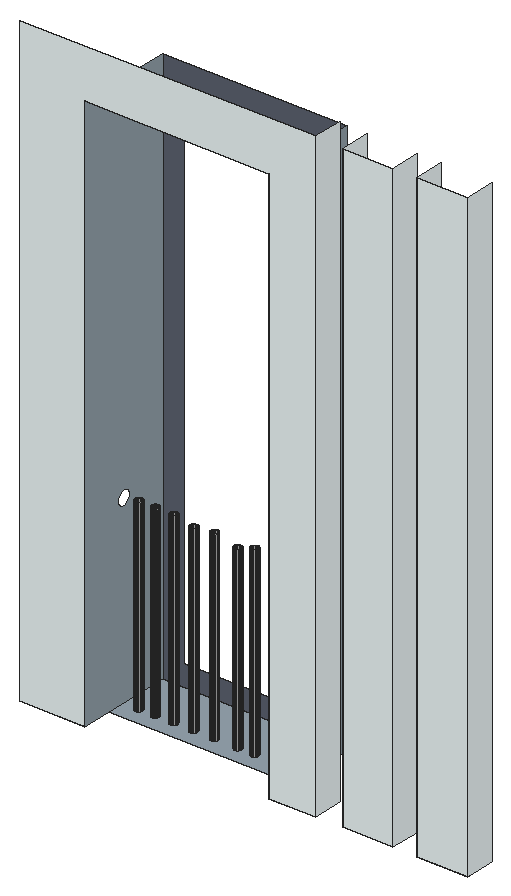
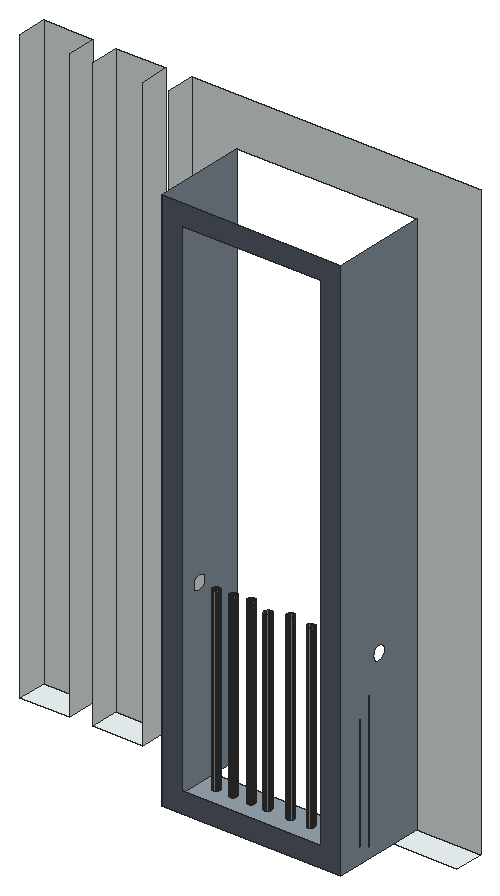
# SketchUp Ruby script. Lengths in inches.
U = 1.inch
M = Sketchup.active_model
def pt(a) = Geom::Point3d.new(a.map { |v| v * U })
def face(e, loops, mat)
  f = e.add_face(loops[0].map { |a| pt(a) })
  loops[1..].each { |l| e.add_face(l.map { |a| pt(a) }).erase! }
  f.material = f.back_material = mat if mat
  f
end
# faces: each face lists its corners as indices into pts; further lists are holes
def faces(e, pts, list, mat = nil) = list.each { |f| face(e, (f[0].is_a?(Array) ? f : [f]).map { |l| l.map { |i| pts[i] } }, mat) }
# xy, xz, yz: faces in a plane at the given z, y or x. An outline is a flat list of corners, or four numbers for a rectangle; further outlines are holes
def ring(l) = l.size == 4 ? [[l[0], l[1]], [l[2], l[1]], [l[2], l[3]], [l[0], l[3]]] : l.each_slice(2).to_a
def flat(e, list, mat, &to3) = list.each { |f| face(e, (f[0].is_a?(Array) ? f : [f]).map { |l| ring(l).map { |u, v| to3.(u, v) } }, mat) }
def xy(e, z, list, mat = nil) = flat(e, list, mat) { |x, y| [x, y, z] }
def xz(e, y, list, mat = nil) = flat(e, list, mat) { |x, z| [x, y, z] }
def yz(e, x, list, mat = nil) = flat(e, list, mat) { |y, z| [x, y, z] }
def lines(e, pts, list) = list.each { |a, b| e.add_line(pt(pts[a]), pt(pts[b])) }
# prism: a flat outline (further loops are holes) pulled along v
def prism(e, loops, v, mat = nil)
  f = face(e, loops, mat); d = Geom::Vector3d.new(v.map { |x| x * U })
  f.pushpull(f.normal.samedirection?(d) ? d.length : -d.length)
end
def box(e, o, s, mat = nil) = prism(e, [[o, [o[0] + s[0], o[1], o[2]], [o[0] + s[0], o[1] + s[1], o[2]], [o[0], o[1] + s[1], o[2]]]], [0, 0, s[2]], mat)
def at(x, y, z, deg = 0) = Geom::Transformation.translation(pt([x, y, z])) * Geom::Transformation.rotation(ORIGIN, Z_AXIS, deg.degrees)
def axes(o, x, y, z) = Geom::Transformation.new([*x, 0, *y, 0, *z, 0, *pt(o).to_a, 1])
def part(name) = M.definitions.add(name)
# library, detail: a bought-in or finely detailed component or shape, given as its bounding box
def library(name, o, s) = part(name).tap { |d| box(d.entities, o, s) }
def detail(e, o, s) = box(e.add_group.entities, o, s)
def put(e, d, t, mat = nil) = e.add_instance(d, t).tap { |i| i.material = mat if mat }
def group(e, t, mat = nil) = e.add_group.tap { |g| g.transformation = t; g.material = mat if mat }.entities
root = M.entities
M.materials.add("[Color M03]").color = [170, 170, 170]
M.materials.add("[Formica Laminate Dark]").color = [95, 101, 114]
M.materials.add("[Terrazzo Light Blue]").color = [151, 165, 175]
M.materials.add("[White Subway Tile]").color = [243, 252, 253]
xy(root,1217.33,[[1131.58,820.58,1130.43,820.73,1129.36,821.17,1128.44,821.88,1127.74,822.8,1127.29,823.87,1127.14,825.02,1127.29,826.17,1127.74,827.24,1128.44,828.15,1129.36,828.86,1130.43,829.3,1131.58,829.45,1132.73,829.3,1133.8,828.86,1134.72,828.15,1135.42,827.24,1135.87,826.17,1136.02,825.02,1135.87,823.87,1135.42,822.8,1134.72,821.88,1133.8,821.17,1132.73,820.73],[1151.52,820.58,1150.37,820.73,1149.3,821.17,1148.38,821.88,1147.67,822.8,1147.23,823.87,1147.08,825.02,1147.23,826.17,1147.67,827.24,1148.38,828.15,1149.3,828.86,1150.37,829.3,1151.52,829.45,1152.67,829.3,1153.74,828.86,1154.65,828.15,1155.36,827.24,1155.8,826.17,1155.95,825.02,1155.8,823.87,1155.36,822.8,1154.65,821.88,1153.74,821.17,1152.67,820.73],[1173.58,820.58,1172.43,820.73,1171.36,821.17,1170.44,821.88,1169.74,822.8,1169.29,823.87,1169.14,825.02,1169.29,826.17,1169.74,827.24,1170.44,828.15,1171.36,828.86,1172.43,829.3,1173.58,829.45,1174.73,829.3,1175.8,828.86,1176.72,828.15,1177.42,827.24,1177.87,826.17,1178.02,825.02,1177.87,823.87,1177.42,822.8,1176.72,821.88,1175.8,821.17,1174.73,820.73],[1197.58,820.58,1196.43,820.73,1195.36,821.17,1194.44,821.88,1193.74,822.8,1193.29,823.87,1193.14,825.02,1193.29,826.17,1193.74,827.24,1194.44,828.15,1195.36,828.86,1196.43,829.3,1197.58,829.45,1198.73,829.3,1199.8,828.86,1200.72,828.15,1201.42,827.24,1201.87,826.17,1202.02,825.02,1201.87,823.87,1201.42,822.8,1200.72,821.88,1199.8,821.17,1198.73,820.73],[1222.58,820.58,1221.43,820.73,1220.36,821.17,1219.44,821.88,1218.74,822.8,1218.29,823.87,1218.14,825.02,1218.29,826.17,1218.74,827.24,1219.44,828.15,1220.36,828.86,1221.43,829.3,1222.58,829.45,1223.73,829.3,1224.8,828.86,1225.72,828.15,1226.42,827.24,1226.87,826.17,1227.02,825.02,1226.87,823.87,1226.42,822.8,1225.72,821.88,1224.8,821.17,1223.73,820.73],
  [1250.58,820.58,1249.43,820.73,1248.36,821.17,1247.44,821.88,1246.74,822.8,1246.29,823.87,1246.14,825.02,1246.29,826.17,1246.74,827.24,1247.44,828.15,1248.36,828.86,1249.43,829.3,1250.58,829.45,1251.73,829.3,1252.8,828.86,1253.72,828.15,1254.42,827.24,1254.87,826.17,1255.02,825.02,1254.87,823.87,1254.42,822.8,1253.72,821.88,1252.8,821.17,1251.73,820.73],[1271.08,820.58,1269.93,820.73,1268.86,821.17,1267.94,821.88,1267.24,822.8,1266.79,823.87,1266.64,825.02,1266.79,826.17,1267.24,827.24,1267.94,828.15,1268.86,828.86,1269.93,829.3,1271.08,829.45,1272.23,829.3,1273.3,828.86,1274.22,828.15,1274.92,827.24,1275.37,826.17,1275.52,825.02,1275.37,823.87,1274.92,822.8,1274.22,821.88,1273.3,821.17,1272.23,820.73],[1292.95,820.58,1291.81,820.73,1290.74,821.17,1289.82,821.88,1289.11,822.8,1288.67,823.87,1288.52,825.02,1288.67,826.17,1289.11,827.24,1289.82,828.15,1290.74,828.86,1291.81,829.3,1292.95,829.45,1294.1,829.3,1295.17,828.86,1296.09,828.15,1296.8,827.24,1297.24,826.17,1297.39,825.02,1297.24,823.87,1296.8,822.8,1296.09,821.88,1295.17,821.17,1294.1,820.73],[1314.2,820.58,1313.06,820.73,1311.99,821.17,1311.07,821.88,1310.36,822.8,1309.92,823.87,1309.77,825.02,1309.92,826.17,1310.36,827.24,1311.07,828.15,1311.99,828.86,1313.06,829.3,1314.2,829.45,1315.35,829.3,1316.42,828.86,1317.34,828.15,1318.05,827.24,1318.49,826.17,1318.64,825.02,1318.49,823.87,1318.05,822.8,1317.34,821.88,1316.42,821.17,1315.35,820.73]])
xy(root,1217.33,[[[1113.04,803.71,1334.04,884.27],[1131.58,820.58,1130.43,820.73,1129.36,821.17,1128.44,821.88,1127.74,822.8,1127.29,823.87,1127.14,825.02,1127.29,826.17,1127.74,827.24,1128.44,828.15,1129.36,828.86,1130.43,829.3,1131.58,829.45,1132.73,829.3,1133.8,828.86,1134.72,828.15,1135.42,827.24,1135.87,826.17,1136.02,825.02,1135.87,823.87,1135.42,822.8,1134.72,821.88,1133.8,821.17,1132.73,820.73],[1314.2,820.58,1313.06,820.73,1311.99,821.17,1311.07,821.88,1310.36,822.8,1309.92,823.87,1309.77,825.02,1309.92,826.17,1310.36,827.24,1311.07,828.15,1311.99,828.86,1313.06,829.3,1314.2,829.45,1315.35,829.3,1316.42,828.86,1317.34,828.15,1318.05,827.24,1318.49,826.17,1318.64,825.02,1318.49,823.87,1318.05,822.8,1317.34,821.88,1316.42,821.17,1315.35,820.73],[1151.52,820.58,1150.37,820.73,1149.3,821.17,1148.38,821.88,1147.67,822.8,1147.23,823.87,1147.08,825.02,1147.23,826.17,1147.67,827.24,1148.38,828.15,1149.3,828.86,1150.37,829.3,1151.52,829.45,1152.67,829.3,1153.74,828.86,1154.65,828.15,1155.36,827.24,1155.8,826.17,1155.95,825.02,1155.8,823.87,1155.36,822.8,1154.65,821.88,1153.74,821.17,1152.67,820.73],[1292.95,820.58,1291.81,820.73,1290.74,821.17,1289.82,821.88,1289.11,822.8,1288.67,823.87,1288.52,825.02,1288.67,826.17,1289.11,827.24,1289.82,828.15,1290.74,828.86,1291.81,829.3,1292.95,829.45,1294.1,829.3,1295.17,828.86,1296.09,828.15,1296.8,827.24,1297.24,826.17,1297.39,825.02,1297.24,823.87,1296.8,822.8,1296.09,821.88,1295.17,821.17,1294.1,820.73],[1173.58,820.58,1172.43,820.73,1171.36,821.17,1170.44,821.88,1169.74,822.8,1169.29,823.87,1169.14,825.02,1169.29,826.17,1169.74,827.24,1170.44,828.15,1171.36,828.86,1172.43,829.3,1173.58,829.45,1174.73,829.3,1175.8,828.86,1176.72,828.15,1177.42,827.24,1177.87,826.17,1178.02,825.02,1177.87,823.87,1177.42,822.8,1176.72,821.88,1175.8,821.17,1174.73,820.73],[1271.08,820.58,1269.93,820.73,1268.86,821.17,1267.94,821.88,1267.24,822.8,1266.79,823.87,1266.64,825.02,1266.79,826.17,1267.24,827.24,1267.94,828.15,1268.86,828.86,1269.93,829.3,1271.08,829.45,1272.23,829.3,1273.3,828.86,1274.22,828.15,1274.92,827.24,1275.37,826.17,1275.52,825.02,1275.37,823.87,1274.92,822.8,1274.22,821.88,1273.3,821.17,1272.23,820.73],[1197.58,820.58,1196.43,820.73,1195.36,821.17,1194.44,821.88,1193.74,822.8,1193.29,823.87,1193.14,825.02,1193.29,826.17,1193.74,827.24,1194.44,828.15,1195.36,828.86,1196.43,829.3,1197.58,829.45,1198.73,829.3,1199.8,828.86,1200.72,828.15,1201.42,827.24,1201.87,826.17,1202.02,825.02,1201.87,823.87,1201.42,822.8,1200.72,821.88,1199.8,821.17,1198.73,820.73],[1250.58,820.58,1249.43,820.73,1248.36,821.17,1247.44,821.88,1246.74,822.8,1246.29,823.87,1246.14,825.02,1246.29,826.17,1246.74,827.24,1247.44,828.15,1248.36,828.86,1249.43,829.3,1250.58,829.45,1251.73,829.3,1252.8,828.86,1253.72,828.15,1254.42,827.24,1254.87,826.17,1255.02,825.02,1254.87,823.87,1254.42,822.8,1253.72,821.88,1252.8,821.17,1251.73,820.73],[1222.58,820.58,1221.43,820.73,1220.36,821.17,1219.44,821.88,1218.74,822.8,1218.29,823.87,1218.14,825.02,1218.29,826.17,1218.74,827.24,1219.44,828.15,1220.36,828.86,1221.43,829.3,1222.58,829.45,1223.73,829.3,1224.8,828.86,1225.72,828.15,1226.42,827.24,1226.87,826.17,1227.02,825.02,1226.87,823.87,1226.42,822.8,1225.72,821.88,1224.8,821.17,1223.73,820.73]]],"[Terrazzo Light Blue]")
xy(root,1217.33,[[1034.97,767.89,1113.04,803.71],[1334.04,767.89,1389.66,803.71]],"[White Subway Tile]")
xy(root,1217.36,[[1421.94,767.89,1482.63,803.71],[1511.44,767.89,1572.13,803.71]],"[White Subway Tile]")
xz(root,767.89,[[1034.97,1217.33,1113.04,1217.33,1113.04,1889.95,1334.04,1889.95,1334.04,1217.33,1389.66,1217.33,1389.66,1949.53,1034.97,1949.53],[1421.94,1217.36,1482.63,1947.36],[1511.44,1217.36,1572.13,1947.36]],"[White Subway Tile]")
xz(root,884.27,[[[1113.04,1217.33,1334.04,1889.95],[1137.95,1242.25,1309.12,1865.04]]],"[Formica Laminate Dark]")
yz(root,1113.04,[[[767.89,1217.33,884.27,1889.95],[826.07,1428.86,823.76,1429.16,821.6,1430.06,819.75,1431.48,818.33,1433.33,817.4375,1435.48,817.13,1437.8,817.4375,1440.11,818.33,1442.27,819.75,1444.12,821.6,1445.54,823.76,1446.43,826.07,1446.73,828.38,1446.43,830.54,1445.54,832.39,1444.12,833.8125,1442.27,834.7,1440.11,835.01,1437.8,834.7,1435.48,833.8125,1433.33,832.39,1431.48,830.54,1430.06,828.38,1429.16]]],"[Terrazzo Light Blue]")
yz(root,1334.04,[[[767.89,1217.33,884.27,1889.95],[826.07,1428.86,828.38,1429.16,830.54,1430.06,832.39,1431.48,833.8125,1433.33,834.7,1435.48,835.01,1437.8,834.7,1440.11,833.8125,1442.27,832.39,1444.12,830.54,1445.54,828.38,1446.43,826.07,1446.73,823.76,1446.43,821.6,1445.54,819.75,1444.12,818.33,1442.27,817.4375,1440.11,817.13,1437.8,817.4375,1435.48,818.33,1433.33,819.75,1431.48,821.6,1430.06,823.76,1429.16]]],"[Terrazzo Light Blue]")
yz(root,1389.66,[[767.89,1217.33,803.71,1949.53]],"[White Subway Tile]")
yz(root,1421.94,[[767.89,1217.36,803.71,1947.36]],"[White Subway Tile]")
yz(root,1482.63,[[767.89,1217.36,803.71,1947.36]],"[White Subway Tile]")
yz(root,1511.44,[[767.89,1217.36,803.71,1947.36]],"[White Subway Tile]")
yz(root,1572.13,[[767.89,1217.36,803.71,1947.36]],"[White Subway Tile]")
p = [[1130.43,820.73,1217.33],[1131.58,820.58,1217.33],[1131.58,820.58,1442.27],[1130.43,820.73,1442.27],[1132.73,820.73,1217.33],[1132.73,820.73,1442.27],
  [1150.37,820.73,1217.33],[1151.52,820.58,1217.33],[1151.52,820.58,1442.27],[1150.37,820.73,1442.27],[1152.67,820.73,1217.33],[1152.67,820.73,1442.27],
  [1172.43,820.73,1217.33],[1173.58,820.58,1217.33],[1173.58,820.58,1442.27],[1172.43,820.73,1442.27],[1174.73,820.73,1217.33],[1174.73,820.73,1442.27],
  [1196.43,820.73,1217.33],[1197.58,820.58,1217.33],[1197.58,820.58,1437.08],[1196.43,820.73,1437.08],[1198.73,820.73,1217.33],[1198.73,820.73,1437.08],
  [1221.43,820.73,1217.33],[1222.58,820.58,1217.33],[1222.58,820.58,1440.11],[1221.43,820.73,1440.11],[1223.73,820.73,1217.33],[1223.73,820.73,1440.11],
  [1249.43,820.73,1217.33],[1250.58,820.58,1217.33],[1250.58,820.58,1433.45],[1249.43,820.73,1433.45],[1251.73,820.73,1217.33],[1251.73,820.73,1433.45],
  [1269.93,820.73,1217.33],[1271.08,820.58,1217.33],[1271.08,820.58,1440.11],[1269.93,820.73,1440.11],[1272.23,820.73,1217.33],[1272.23,820.73,1440.11],
  [1291.81,820.73,1217.33],[1292.95,820.58,1217.33],[1292.95,820.58,1437.8],[1291.81,820.73,1437.8],[1294.1,820.73,1217.33],[1294.1,820.73,1437.8],
  [1313.06,820.73,1217.33],[1314.2,820.58,1217.33],[1314.2,820.58,1436.77],[1313.06,820.73,1436.77],[1315.35,820.73,1217.33],[1315.35,820.73,1436.77],
  [1129.36,821.17,1217.33],[1129.36,821.17,1442.27],[1133.8,821.17,1217.33],[1133.8,821.17,1442.27],[1149.3,821.17,1217.33],[1149.3,821.17,1442.27],
  [1153.74,821.17,1217.33],[1153.74,821.17,1442.27],[1171.36,821.17,1217.33],[1171.36,821.17,1442.27],[1175.8,821.17,1217.33],[1175.8,821.17,1442.27],
  [1195.36,821.17,1217.33],[1195.36,821.17,1437.08],[1199.8,821.17,1217.33],[1199.8,821.17,1437.08],[1220.36,821.17,1217.33],[1220.36,821.17,1440.11],
  [1224.8,821.17,1217.33],[1224.8,821.17,1440.11],[1248.36,821.17,1217.33],[1248.36,821.17,1433.45],[1252.8,821.17,1217.33],[1252.8,821.17,1433.45],
  [1268.86,821.17,1217.33],[1268.86,821.17,1440.11],[1273.3,821.17,1217.33],[1273.3,821.17,1440.11],[1290.74,821.17,1217.33],[1290.74,821.17,1437.8],
  [1295.17,821.17,1217.33],[1295.17,821.17,1437.8],[1311.99,821.17,1217.33],[1311.99,821.17,1436.77],[1316.42,821.17,1217.33],[1316.42,821.17,1436.77],
  [1128.44,821.88,1217.33],[1128.44,821.88,1442.27],[1134.72,821.88,1217.33],[1134.72,821.88,1442.27],[1148.38,821.88,1217.33],[1148.38,821.88,1442.27],
  [1154.65,821.88,1217.33],[1154.65,821.88,1442.27],[1170.44,821.88,1217.33],[1170.44,821.88,1442.27],[1176.72,821.88,1217.33],[1176.72,821.88,1442.27],
  [1194.44,821.88,1217.33],[1194.44,821.88,1437.08],[1200.72,821.88,1217.33],[1200.72,821.88,1437.08],[1219.44,821.88,1217.33],[1219.44,821.88,1440.11],
  [1225.72,821.88,1217.33],[1225.72,821.88,1440.11],[1247.44,821.88,1217.33],[1247.44,821.88,1433.45],[1253.72,821.88,1217.33],[1253.72,821.88,1433.45],
  [1267.94,821.88,1217.33],[1267.94,821.88,1440.11],[1274.22,821.88,1217.33],[1274.22,821.88,1440.11],[1289.82,821.88,1217.33],[1289.82,821.88,1437.8],
  [1296.09,821.88,1217.33],[1296.09,821.88,1437.8],[1311.07,821.88,1217.33],[1311.07,821.88,1436.77],[1317.34,821.88,1217.33],[1317.34,821.88,1436.77],
  [1127.74,822.8,1217.33],[1127.74,822.8,1442.27],[1135.42,822.8,1217.33],[1135.42,822.8,1442.27],[1147.67,822.8,1217.33],[1147.67,822.8,1442.27],
  [1155.36,822.8,1217.33],[1155.36,822.8,1442.27],[1169.74,822.8,1217.33],[1169.74,822.8,1442.27],[1177.42,822.8,1217.33],[1177.42,822.8,1442.27],
  [1193.74,822.8,1217.33],[1193.74,822.8,1437.08],[1201.42,822.8,1217.33],[1201.42,822.8,1437.08],[1218.74,822.8,1217.33],[1218.74,822.8,1440.11],
  [1226.42,822.8,1217.33],[1226.42,822.8,1440.11],[1246.74,822.8,1217.33],[1246.74,822.8,1433.45],[1254.42,822.8,1217.33],[1254.42,822.8,1433.45],
  [1267.24,822.8,1217.33],[1267.24,822.8,1440.11],[1274.92,822.8,1217.33],[1274.92,822.8,1440.11],[1289.11,822.8,1217.33],[1289.11,822.8,1437.8],
  [1296.8,822.8,1217.33],[1296.8,822.8,1437.8],[1310.36,822.8,1217.33],[1310.36,822.8,1436.77],[1318.05,822.8,1217.33],[1318.05,822.8,1436.77],
  [1127.29,823.87,1217.33],[1127.29,823.87,1442.27],[1135.87,823.87,1217.33],[1135.87,823.87,1442.27],[1147.23,823.87,1217.33],[1147.23,823.87,1442.27],
  [1155.8,823.87,1217.33],[1155.8,823.87,1442.27],[1169.29,823.87,1217.33],[1169.29,823.87,1442.27],[1177.87,823.87,1217.33],[1177.87,823.87,1442.27],
  [1193.29,823.87,1217.33],[1193.29,823.87,1437.08],[1201.87,823.87,1217.33],[1201.87,823.87,1437.08],[1218.29,823.87,1217.33],[1218.29,823.87,1440.11],
  [1226.87,823.87,1217.33],[1226.87,823.87,1440.11],[1246.29,823.87,1217.33],[1246.29,823.87,1433.45],[1254.87,823.87,1217.33],[1254.87,823.87,1433.45],
  [1266.79,823.87,1217.33],[1266.79,823.87,1440.11],[1275.37,823.87,1217.33],[1275.37,823.87,1440.11],[1288.67,823.87,1217.33],[1288.67,823.87,1437.8],
  [1297.24,823.87,1217.33],[1297.24,823.87,1437.8],[1309.92,823.87,1217.33],[1309.92,823.87,1436.77],[1318.49,823.87,1217.33],[1318.49,823.87,1436.77],
  [1127.14,825.02,1217.33],[1127.14,825.02,1442.27],[1136.02,825.02,1217.33],[1136.02,825.02,1442.27],[1147.08,825.02,1217.33],[1147.08,825.02,1442.27],
  [1155.95,825.02,1217.33],[1155.95,825.02,1442.27],[1169.14,825.02,1217.33],[1169.14,825.02,1442.27],[1178.02,825.02,1217.33],[1178.02,825.02,1442.27],
  [1193.14,825.02,1217.33],[1193.14,825.02,1437.08],[1202.02,825.02,1217.33],[1202.02,825.02,1437.08],[1218.14,825.02,1217.33],[1218.14,825.02,1440.11],
  [1227.02,825.02,1217.33],[1227.02,825.02,1440.11],[1246.14,825.02,1217.33],[1246.14,825.02,1433.45],[1255.02,825.02,1217.33],[1255.02,825.02,1433.45],
  [1266.64,825.02,1217.33],[1266.64,825.02,1440.11],[1275.52,825.02,1217.33],[1275.52,825.02,1440.11],[1288.52,825.02,1217.33],[1288.52,825.02,1437.8],
  [1297.39,825.02,1217.33],[1297.39,825.02,1437.8],[1309.77,825.02,1217.33],[1309.77,825.02,1436.77],[1318.64,825.02,1217.33],[1318.64,825.02,1436.77],
  [1127.29,826.17,1217.33],[1127.29,826.17,1442.27],[1135.87,826.17,1217.33],[1135.87,826.17,1442.27],[1147.23,826.17,1217.33],[1147.23,826.17,1442.27],
  [1155.8,826.17,1217.33],[1155.8,826.17,1442.27],[1169.29,826.17,1217.33],[1169.29,826.17,1442.27],[1177.87,826.17,1217.33],[1177.87,826.17,1442.27],
  [1193.29,826.17,1217.33],[1193.29,826.17,1437.08],[1201.87,826.17,1217.33],[1201.87,826.17,1437.08],[1218.29,826.17,1217.33],[1218.29,826.17,1440.11],
  [1226.87,826.17,1217.33],[1226.87,826.17,1440.11],[1246.29,826.17,1217.33],[1246.29,826.17,1433.45],[1254.87,826.17,1217.33],[1254.87,826.17,1433.45],
  [1266.79,826.17,1217.33],[1266.79,826.17,1440.11],[1275.37,826.17,1217.33],[1275.37,826.17,1440.11],[1288.67,826.17,1217.33],[1288.67,826.17,1437.8],
  [1297.24,826.17,1217.33],[1297.24,826.17,1437.8],[1309.92,826.17,1217.33],[1309.92,826.17,1436.77],[1318.49,826.17,1217.33],[1318.49,826.17,1436.77],
  [1127.74,827.24,1217.33],[1127.74,827.24,1442.27],[1135.42,827.24,1217.33],[1135.42,827.24,1442.27],[1147.67,827.24,1217.33],[1147.67,827.24,1442.27],
  [1155.36,827.24,1217.33],[1155.36,827.24,1442.27],[1169.74,827.24,1217.33],[1169.74,827.24,1442.27],[1177.42,827.24,1217.33],[1177.42,827.24,1442.27],
  [1193.74,827.24,1217.33],[1193.74,827.24,1437.08],[1201.42,827.24,1217.33],[1201.42,827.24,1437.08],[1218.74,827.24,1217.33],[1218.74,827.24,1440.11],
  [1226.42,827.24,1217.33],[1226.42,827.24,1440.11],[1246.74,827.24,1217.33],[1246.74,827.24,1433.45],[1254.42,827.24,1217.33],[1254.42,827.24,1433.45],
  [1267.24,827.24,1217.33],[1267.24,827.24,1440.11],[1274.92,827.24,1217.33],[1274.92,827.24,1440.11],[1289.11,827.24,1217.33],[1289.11,827.24,1437.8],
  [1296.8,827.24,1217.33],[1296.8,827.24,1437.8],[1310.36,827.24,1217.33],[1310.36,827.24,1436.77],[1318.05,827.24,1217.33],[1318.05,827.24,1436.77],
  [1128.44,828.15,1217.33],[1128.44,828.15,1442.27],[1134.72,828.15,1217.33],[1134.72,828.15,1442.27],[1148.38,828.15,1217.33],[1148.38,828.15,1442.27],
  [1154.65,828.15,1217.33],[1154.65,828.15,1442.27],[1170.44,828.15,1217.33],[1170.44,828.15,1442.27],[1176.72,828.15,1217.33],[1176.72,828.15,1442.27],
  [1194.44,828.15,1217.33],[1194.44,828.15,1437.08],[1200.72,828.15,1217.33],[1200.72,828.15,1437.08],[1219.44,828.15,1217.33],[1219.44,828.15,1440.11],
  [1225.72,828.15,1217.33],[1225.72,828.15,1440.11],[1247.44,828.15,1217.33],[1247.44,828.15,1433.45],[1253.72,828.15,1217.33],[1253.72,828.15,1433.45],
  [1267.94,828.15,1217.33],[1267.94,828.15,1440.11],[1274.22,828.15,1217.33],[1274.22,828.15,1440.11],[1289.82,828.15,1217.33],[1289.82,828.15,1437.8],
  [1296.09,828.15,1217.33],[1296.09,828.15,1437.8],[1311.07,828.15,1217.33],[1311.07,828.15,1436.77],[1317.34,828.15,1217.33],[1317.34,828.15,1436.77],
  [1129.36,828.86,1217.33],[1129.36,828.86,1442.27],[1133.8,828.86,1217.33],[1133.8,828.86,1442.27],[1149.3,828.86,1217.33],[1149.3,828.86,1442.27],
  [1153.74,828.86,1217.33],[1153.74,828.86,1442.27],[1171.36,828.86,1217.33],[1171.36,828.86,1442.27],[1175.8,828.86,1217.33],[1175.8,828.86,1442.27],
  [1195.36,828.86,1217.33],[1195.36,828.86,1437.08],[1199.8,828.86,1217.33],[1199.8,828.86,1437.08],[1220.36,828.86,1217.33],[1220.36,828.86,1440.11],
  [1224.8,828.86,1217.33],[1224.8,828.86,1440.11],[1248.36,828.86,1217.33],[1248.36,828.86,1433.45],[1252.8,828.86,1217.33],[1252.8,828.86,1433.45],
  [1268.86,828.86,1217.33],[1268.86,828.86,1440.11],[1273.3,828.86,1217.33],[1273.3,828.86,1440.11],[1290.74,828.86,1217.33],[1290.74,828.86,1437.8],
  [1295.17,828.86,1217.33],[1295.17,828.86,1437.8],[1311.99,828.86,1217.33],[1311.99,828.86,1436.77],[1316.42,828.86,1217.33],[1316.42,828.86,1436.77],
  [1130.43,829.3,1217.33],[1130.43,829.3,1442.27],[1132.73,829.3,1217.33],[1132.73,829.3,1442.27],[1150.37,829.3,1217.33],[1150.37,829.3,1442.27],
  [1152.67,829.3,1217.33],[1152.67,829.3,1442.27],[1172.43,829.3,1217.33],[1172.43,829.3,1442.27],[1174.73,829.3,1217.33],[1174.73,829.3,1442.27],
  [1196.43,829.3,1217.33],[1196.43,829.3,1437.08],[1198.73,829.3,1217.33],[1198.73,829.3,1437.08],[1221.43,829.3,1217.33],[1221.43,829.3,1440.11],
  [1223.73,829.3,1217.33],[1223.73,829.3,1440.11],[1249.43,829.3,1217.33],[1249.43,829.3,1433.45],[1251.73,829.3,1217.33],[1251.73,829.3,1433.45],
  [1269.93,829.3,1217.33],[1269.93,829.3,1440.11],[1272.23,829.3,1217.33],[1272.23,829.3,1440.11],[1291.81,829.3,1217.33],[1291.81,829.3,1437.8],
  [1294.1,829.3,1217.33],[1294.1,829.3,1437.8],[1313.06,829.3,1217.33],[1313.06,829.3,1436.77],[1315.35,829.3,1217.33],[1315.35,829.3,1436.77],
  [1131.58,829.45,1217.33],[1131.58,829.45,1442.27],[1151.52,829.45,1217.33],[1151.52,829.45,1442.27],[1173.58,829.45,1217.33],[1173.58,829.45,1442.27],
  [1197.58,829.45,1217.33],[1197.58,829.45,1437.08],[1222.58,829.45,1217.33],[1222.58,829.45,1440.11],[1250.58,829.45,1217.33],[1250.58,829.45,1433.45],
  [1271.08,829.45,1217.33],[1271.08,829.45,1440.11],[1292.95,829.45,1217.33],[1292.95,829.45,1437.8],[1314.2,829.45,1217.33],[1314.2,829.45,1436.77]]
faces(root,p,[[0,1,2,3],[1,4,5,2],[6,7,8,9],[7,10,11,8],[12,13,14,15],[13,16,17,14],[18,19,20,21],[19,22,23,20],
  [24,25,26,27],[25,28,29,26],[30,31,32,33],[31,34,35,32],[36,37,38,39],[37,40,41,38],[42,43,44,45],[43,46,47,44],
  [48,49,50,51],[49,52,53,50],[54,0,3,55],[4,56,57,5],[58,6,9,59],[10,60,61,11],[62,12,15,63],[16,64,65,17],
  [66,18,21,67],[22,68,69,23],[70,24,27,71],[28,72,73,29],[74,30,33,75],[34,76,77,35],[78,36,39,79],[40,80,81,41],
  [82,42,45,83],[46,84,85,47],[86,48,51,87],[52,88,89,53],[90,54,55,91],[56,92,93,57],[94,58,59,95],[60,96,97,61],
  [98,62,63,99],[64,100,101,65],[102,66,67,103],[68,104,105,69],[106,70,71,107],[72,108,109,73],[110,74,75,111],[76,112,113,77],
  [114,78,79,115],[80,116,117,81],[118,82,83,119],[84,120,121,85],[122,86,87,123],[88,124,125,89],[126,90,91,127],[92,128,129,93],
  [130,94,95,131],[96,132,133,97],[134,98,99,135],[100,136,137,101],[138,102,103,139],[104,140,141,105],[142,106,107,143],[108,144,145,109],
  [146,110,111,147],[112,148,149,113],[150,114,115,151],[116,152,153,117],[154,118,119,155],[120,156,157,121],[158,122,123,159],[124,160,161,125],
  [162,126,127,163],[128,164,165,129],[166,130,131,167],[132,168,169,133],[170,134,135,171],[136,172,173,137],[174,138,139,175],[140,176,177,141],
  [178,142,143,179],[144,180,181,145],[182,146,147,183],[148,184,185,149],[186,150,151,187],[152,188,189,153],[190,154,155,191],[156,192,193,157],
  [194,158,159,195],[160,196,197,161],[198,162,163,199],[164,200,201,165],[202,166,167,203],[168,204,205,169],[206,170,171,207],[172,208,209,173],
  [210,174,175,211],[176,212,213,177],[214,178,179,215],[180,216,217,181],[218,182,183,219],[184,220,221,185],[222,186,187,223],[188,224,225,189],
  [226,190,191,227],[192,228,229,193],[230,194,195,231],[196,232,233,197],[234,198,199,235],[200,236,237,201],[238,202,203,239],[204,240,241,205],
  [242,206,207,243],[208,244,245,209],[246,210,211,247],[212,248,249,213],[250,214,215,251],[216,252,253,217],[254,218,219,255],[220,256,257,221],
  [258,222,223,259],[224,260,261,225],[262,226,227,263],[228,264,265,229],[266,230,231,267],[232,268,269,233],[270,234,235,271],[236,272,273,237],
  [274,238,239,275],[240,276,277,241],[278,242,243,279],[244,280,281,245],[282,246,247,283],[248,284,285,249],[286,250,251,287],[252,288,289,253],
  [290,254,255,291],[256,292,293,257],[294,258,259,295],[260,296,297,261],[298,262,263,299],[264,300,301,265],[302,266,267,303],[268,304,305,269],
  [306,270,271,307],[272,308,309,273],[310,274,275,311],[276,312,313,277],[314,278,279,315],[280,316,317,281],[318,282,283,319],[284,320,321,285],
  [322,286,287,323],[288,324,325,289],[326,290,291,327],[292,328,329,293],[330,294,295,331],[296,332,333,297],[334,298,299,335],[300,336,337,301],
  [338,302,303,339],[304,340,341,305],[342,306,307,343],[308,344,345,309],[346,310,311,347],[312,348,349,313],[350,314,315,351],[316,352,353,317],
  [354,318,319,355],[320,356,357,321],[358,322,323,359],[324,360,361,325],[362,326,327,363],[328,364,365,329],[366,330,331,367],[332,368,369,333],
  [370,334,335,371],[336,372,373,337],[374,338,339,375],[340,376,377,341],[378,342,343,379],[344,380,381,345],[382,346,347,383],[348,384,385,349],
  [386,350,351,387],[352,388,389,353],[390,354,355,391],[356,392,393,357],[394,358,359,395],[360,396,397,361],[398,362,363,399],[364,400,401,365],
  [402,366,367,403],[368,404,405,369],[406,370,371,407],[372,408,409,373],[410,374,375,411],[376,412,413,377],[414,378,379,415],[380,414,415,381],
  [416,382,383,417],[384,416,417,385],[418,386,387,419],[388,418,419,389],[420,390,391,421],[392,420,421,393],[422,394,395,423],[396,422,423,397],
  [424,398,399,425],[400,424,425,401],[426,402,403,427],[404,426,427,405],[428,406,407,429],[408,428,429,409],[430,410,411,431],[412,430,431,413]],"[Color M03]")
